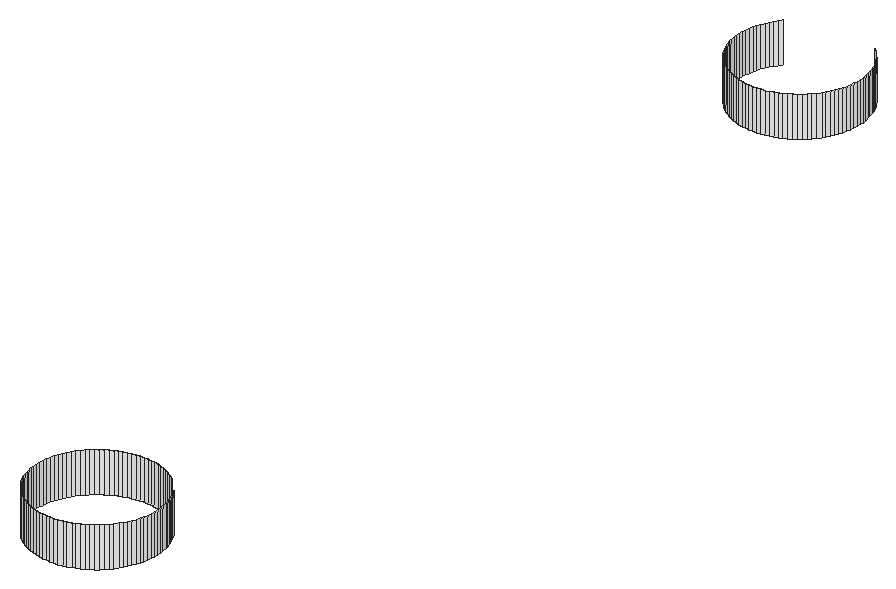
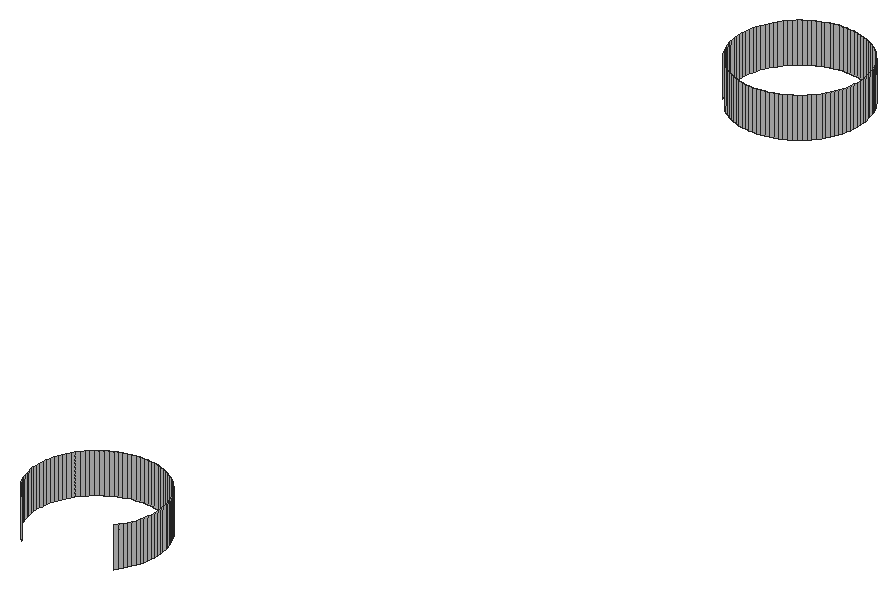
# SketchUp Ruby script. Lengths in inches.
U = 1.inch
M = Sketchup.active_model
def pt(a) = Geom::Point3d.new(a.map { |v| v * U })
def face(e, loops, mat)
  f = e.add_face(loops[0].map { |a| pt(a) })
  loops[1..].each { |l| e.add_face(l.map { |a| pt(a) }).erase! }
  f.material = f.back_material = mat if mat
  f
end
# faces: each face lists its corners as indices into pts; further lists are holes
def faces(e, pts, list, mat = nil) = list.each { |f| face(e, (f[0].is_a?(Array) ? f : [f]).map { |l| l.map { |i| pts[i] } }, mat) }
# xy, xz, yz: faces in a plane at the given z, y or x. An outline is a flat list of corners, or four numbers for a rectangle; further outlines are holes
def ring(l) = l.size == 4 ? [[l[0], l[1]], [l[2], l[1]], [l[2], l[3]], [l[0], l[3]]] : l.each_slice(2).to_a
def flat(e, list, mat, &to3) = list.each { |f| face(e, (f[0].is_a?(Array) ? f : [f]).map { |l| ring(l).map { |u, v| to3.(u, v) } }, mat) }
def xy(e, z, list, mat = nil) = flat(e, list, mat) { |x, y| [x, y, z] }
def xz(e, y, list, mat = nil) = flat(e, list, mat) { |x, z| [x, y, z] }
def yz(e, x, list, mat = nil) = flat(e, list, mat) { |y, z| [x, y, z] }
def lines(e, pts, list) = list.each { |a, b| e.add_line(pt(pts[a]), pt(pts[b])) }
# prism: a flat outline (further loops are holes) pulled along v
def prism(e, loops, v, mat = nil)
  f = face(e, loops, mat); d = Geom::Vector3d.new(v.map { |x| x * U })
  f.pushpull(f.normal.samedirection?(d) ? d.length : -d.length)
end
def box(e, o, s, mat = nil) = prism(e, [[o, [o[0] + s[0], o[1], o[2]], [o[0] + s[0], o[1] + s[1], o[2]], [o[0], o[1] + s[1], o[2]]]], [0, 0, s[2]], mat)
def at(x, y, z, deg = 0) = Geom::Transformation.translation(pt([x, y, z])) * Geom::Transformation.rotation(ORIGIN, Z_AXIS, deg.degrees)
def axes(o, x, y, z) = Geom::Transformation.new([*x, 0, *y, 0, *z, 0, *pt(o).to_a, 1])
def part(name) = M.definitions.add(name)
# library, detail: a bought-in or finely detailed component or shape, given as its bounding box
def library(name, o, s) = part(name).tap { |d| box(d.entities, o, s) }
def detail(e, o, s) = box(e.add_group.entities, o, s)
def put(e, d, t, mat = nil) = e.add_instance(d, t).tap { |i| i.material = mat if mat }
def group(e, t, mat = nil) = e.add_group.tap { |g| g.transformation = t; g.material = mat if mat }.entities
root = M.entities
M.materials.add("[Color M00]").color = [255, 255, 255]
xz(root,61,[[127.87,120,128.0625,122]],"[Color M00]")
xz(root,67,[[127.9375,120,128.13,122]],"[Color M00]")
xz(root,105,[[127.87,120,128.0625,122]],"[Color M00]")
yz(root,125,[[63.9375,120,64.13,122],[107.9375,120,108.13,122]],"[Color M00]")
yz(root,131,[[63.87,120,64.0625,122],[107.87,120,108.0625,122]],"[Color M00]")
p = [[127.5,61.04,120],[127.3125,61.08,120],[127.3125,61.08,122],[127.5,61.04,122],[127.68,61.02,120],[127.68,61.02,122],
  [127.87,61,120],[127.87,61,122],[128.25,61.01,120],[128.0625,61,120],[128.0625,61,122],[128.25,61.01,122],
  [128.4375,61.03,120],[128.4375,61.03,122],[128.62,61.07,120],[128.62,61.07,122],[127.13,61.13,120],[126.95,61.1875,120],
  [126.95,61.1875,122],[127.13,61.13,122],[128.81,61.11,120],[128.81,61.11,122],[128.98,61.17,120],[128.98,61.17,122],
  [126.78,61.26,120],[126.78,61.26,122],[129.16,61.23,120],[129.16,61.23,122],[129.33,61.3125,120],[129.33,61.3125,122],
  [126.61,61.34,120],[126.44,61.43,120],[126.44,61.43,122],[126.61,61.34,122],[129.5,61.4,120],[129.5,61.4,122],
  [126.29,61.54,120],[126.29,61.54,122],[129.66,61.5,120],[129.66,61.5,122],[126.14,61.65,120],[126.14,61.65,122],
  [129.8125,61.61,120],[129.8125,61.61,122],[125.99,61.77,120],[125.99,61.77,122],[129.96,61.73,120],[129.96,61.73,122],
  [130.1,61.86,120],[130.1,61.86,122],[125.86,61.9,120],[125.86,61.9,122],[125.73,62.04,120],[125.73,62.04,122],
  [130.23,61.99,120],[130.23,61.99,122],[125.61,62.1875,120],[125.61,62.1875,122],[130.35,62.14,120],[130.35,62.14,122],
  [130.46,62.29,120],[130.46,62.29,122],[125.5,62.34,120],[125.5,62.34,122],[125.4,62.5,120],[125.4,62.5,122],
  [130.57,62.44,120],[130.57,62.44,122],[130.66,62.61,120],[130.66,62.61,122],[125.3125,62.67,120],[125.3125,62.67,122],
  [130.74,62.78,120],[130.74,62.78,122],[125.23,62.84,120],[125.23,62.84,122],[125.17,63.02,120],[125.17,63.02,122],
  [130.8125,62.95,120],[130.8125,62.95,122],[125.11,63.19,120],[125.11,63.19,122],[130.87,63.13,120],[130.87,63.13,122],
  [130.92,63.3125,120],[130.92,63.3125,122],[125.07,63.38,120],[125.07,63.38,122],[130.96,63.5,120],[130.96,63.5,122],
  [125.03,63.5625,120],[125.03,63.5625,122],[130.98,63.68,120],[130.98,63.68,122],[125.01,63.75,120],[125.01,63.75,122],
  [131,63.87,120],[131,63.87,122],[125,63.9375,120],[125,63.9375,122],[125,64.13,120],[125.02,64.32,120],
  [125.02,64.32,122],[125,64.13,122],[130.99,64.25,120],[131,64.0625,120],[131,64.0625,122],[130.99,64.25,122],
  [130.97,64.4375,120],[130.97,64.4375,122],[125.04,64.5,120],[125.04,64.5,122],[130.93,64.62,120],[130.93,64.62,122],
  [125.08,64.6875,120],[125.08,64.6875,122],[130.89,64.81,120],[130.89,64.81,122],[125.13,64.87,120],[125.13,64.87,122],
  [130.83,64.98,120],[130.83,64.98,122],[125.1875,65.05,120],[125.1875,65.05,122],[125.26,65.22,120],[125.26,65.22,122],
  [130.77,65.16,120],[130.77,65.16,122],[125.34,65.39,120],[125.34,65.39,122],[130.6875,65.33,120],[130.6875,65.33,122],
  [130.6,65.5,120],[130.6,65.5,122],[125.43,65.56,120],[125.43,65.56,122],[130.5,65.66,120],[130.5,65.66,122],
  [125.54,65.71,120],[125.54,65.71,122],[125.65,65.86,120],[125.65,65.86,122],[125.77,66.01,120],[125.77,66.01,122],
  [125.9,66.14,120],[125.9,66.14,122],[126.04,66.27,120],[126.04,66.27,122],[126.1875,66.39,120],[126.1875,66.39,122],
  [126.34,66.5,120],[126.34,66.5,122],[129.71,66.46,120],[129.86,66.35,120],[129.86,66.35,122],[129.71,66.46,122],
  [126.5,66.6,120],[126.5,66.6,122],[129.56,66.57,120],[129.56,66.57,122],[126.67,66.6875,120],[126.67,66.6875,122],
  [129.39,66.66,120],[129.39,66.66,122],[126.84,66.77,120],[126.84,66.77,122],[129.05,66.8125,120],[129.22,66.74,120],
  [129.22,66.74,122],[129.05,66.8125,122],[127.02,66.83,120],[127.02,66.83,122],[127.19,66.89,120],[127.19,66.89,122],
  [128.87,66.87,120],[128.87,66.87,122],[127.38,66.93,120],[127.38,66.93,122],[127.5625,66.97,120],[127.5625,66.97,122],
  [128.5,66.96,120],[128.6875,66.92,120],[128.6875,66.92,122],[128.5,66.96,122],[127.75,66.99,120],[127.75,66.99,122],
  [127.9375,67,120],[127.9375,67,122],[128.13,67,120],[128.32,66.98,120],[128.32,66.98,122],[128.13,67,122],
  [127.5,105.04,120],[127.3125,105.08,120],[127.3125,105.08,122],[127.5,105.04,122],[127.68,105.02,120],[127.68,105.02,122],
  [127.87,105,120],[127.87,105,122],[128.25,105.01,120],[128.0625,105,120],[128.0625,105,122],[128.25,105.01,122],
  [128.4375,105.03,120],[128.4375,105.03,122],[128.62,105.07,120],[128.62,105.07,122],[127.13,105.13,120],[126.95,105.1875,120],
  [126.95,105.1875,122],[127.13,105.13,122],[128.81,105.11,120],[128.81,105.11,122],[128.98,105.17,120],[128.98,105.17,122],
  [126.78,105.26,120],[126.78,105.26,122],[129.16,105.23,120],[129.16,105.23,122],[129.33,105.3125,120],[129.33,105.3125,122],
  [126.61,105.34,120],[126.44,105.43,120],[126.44,105.43,122],[126.61,105.34,122],[129.5,105.4,120],[129.5,105.4,122],
  [126.29,105.54,120],[126.29,105.54,122],[129.66,105.5,120],[129.66,105.5,122],[126.14,105.65,120],[126.14,105.65,122],
  [129.8125,105.61,120],[129.8125,105.61,122],[125.99,105.77,120],[125.99,105.77,122],[129.96,105.73,120],[129.96,105.73,122],
  [130.1,105.86,120],[130.1,105.86,122],[125.86,105.9,120],[125.86,105.9,122],[125.73,106.04,120],[125.73,106.04,122],
  [130.23,105.99,120],[130.23,105.99,122],[125.61,106.1875,120],[125.61,106.1875,122],[130.35,106.14,120],[130.35,106.14,122],
  [130.46,106.29,120],[130.46,106.29,122],[125.5,106.34,120],[125.5,106.34,122],[125.4,106.5,120],[125.4,106.5,122],
  [130.57,106.44,120],[130.57,106.44,122],[130.66,106.61,120],[130.66,106.61,122],[125.3125,106.67,120],[125.3125,106.67,122],
  [130.74,106.78,120],[130.74,106.78,122],[125.23,106.84,120],[125.23,106.84,122],[125.17,107.02,120],[125.17,107.02,122],
  [130.8125,106.95,120],[130.8125,106.95,122],[125.11,107.19,120],[125.11,107.19,122],[130.87,107.13,120],[130.87,107.13,122],
  [130.92,107.3125,120],[130.92,107.3125,122],[125.07,107.38,120],[125.07,107.38,122],[130.96,107.5,120],[130.96,107.5,122],
  [125.03,107.5625,120],[125.03,107.5625,122],[130.98,107.68,120],[130.98,107.68,122],[125.01,107.75,120],[125.01,107.75,122],
  [131,107.87,120],[131,107.87,122],[125,107.9375,120],[125,107.9375,122],[125,108.13,120],[125.02,108.32,120],
  [125.02,108.32,122],[125,108.13,122],[130.99,108.25,120],[131,108.0625,120],[131,108.0625,122],[130.99,108.25,122],
  [130.97,108.4375,120],[130.97,108.4375,122],[125.04,108.5,120],[125.04,108.5,122],[130.93,108.62,120],[130.93,108.62,122],
  [125.08,108.6875,120],[125.08,108.6875,122],[130.89,108.81,120],[130.89,108.81,122],[125.13,108.87,120],[125.13,108.87,122],
  [130.83,108.98,120],[130.83,108.98,122],[125.1875,109.05,120],[125.1875,109.05,122],[125.26,109.22,120],[125.26,109.22,122],
  [130.77,109.16,120],[130.77,109.16,122],[125.34,109.39,120],[125.34,109.39,122],[130.6875,109.33,120],[130.6875,109.33,122],
  [130.6,109.5,120],[130.6,109.5,122],[125.43,109.56,120],[125.43,109.56,122],[130.5,109.66,120],[130.5,109.66,122],
  [125.54,109.71,120],[125.54,109.71,122],[125.65,109.86,120],[125.65,109.86,122],[130.39,109.8125,120],[130.39,109.8125,122],
  [130.27,109.96,120],[130.27,109.96,122],[130.14,110.1,120],[130.14,110.1,122],[130.01,110.23,120],[130.01,110.23,122],
  [129.86,110.35,120],[129.86,110.35,122]]
faces(root,p,[[0,1,2,3],[4,0,3,5],[6,4,5,7],[8,9,10,11],[12,8,11,13],[14,12,13,15],[16,17,18,19],[1,16,19,2],
  [20,14,15,21],[22,20,21,23],[17,24,25,18],[26,22,23,27],[28,26,27,29],[30,31,32,33],[24,30,33,25],[34,28,29,35],
  [31,36,37,32],[38,34,35,39],[36,40,41,37],[42,38,39,43],[40,44,45,41],[46,42,43,47],[48,46,47,49],[44,50,51,45],
  [50,52,53,51],[54,48,49,55],[52,56,57,53],[58,54,55,59],[60,58,59,61],[56,62,63,57],[62,64,65,63],[66,60,61,67],
  [68,66,67,69],[64,70,71,65],[72,68,69,73],[70,74,75,71],[74,76,77,75],[78,72,73,79],[76,80,81,77],[82,78,79,83],
  [84,82,83,85],[80,86,87,81],[88,84,85,89],[86,90,91,87],[92,88,89,93],[90,94,95,91],[96,92,93,97],[94,98,99,95],
  [100,101,102,103],[104,105,106,107],[108,104,107,109],[101,110,111,102],[112,108,109,113],[110,114,115,111],[116,112,113,117],[114,118,119,115],
  [120,116,117,121],[118,122,123,119],[122,124,125,123],[126,120,121,127],[124,128,129,125],[130,126,127,131],[132,130,131,133],[128,134,135,129],
  [136,132,133,137],[134,138,139,135],[138,140,141,139],[140,142,143,141],[142,144,145,143],[144,146,147,145],[146,148,149,147],[148,150,151,149],
  [152,153,154,155],[150,156,157,151],[158,152,155,159],[156,160,161,157],[162,158,159,163],[160,164,165,161],[166,167,168,169],[167,162,163,168],
  [164,170,171,165],[170,172,173,171],[174,166,169,175],[172,176,177,173],[176,178,179,177],[180,181,182,183],[181,174,175,182],[178,184,185,179],
  [184,186,187,185],[188,189,190,191],[189,180,183,190],[192,193,194,195],[196,192,195,197],[198,196,197,199],[200,201,202,203],[204,200,203,205],
  [206,204,205,207],[208,209,210,211],[193,208,211,194],[212,206,207,213],[214,212,213,215],[209,216,217,210],[218,214,215,219],[220,218,219,221],
  [222,223,224,225],[216,222,225,217],[226,220,221,227],[223,228,229,224],[230,226,227,231],[228,232,233,229],[234,230,231,235],[232,236,237,233],
  [238,234,235,239],[240,238,239,241],[236,242,243,237],[242,244,245,243],[246,240,241,247],[244,248,249,245],[250,246,247,251],[252,250,251,253],
  [248,254,255,249],[254,256,257,255],[258,252,253,259],[260,258,259,261],[256,262,263,257],[264,260,261,265],[262,266,267,263],[266,268,269,267],
  [270,264,265,271],[268,272,273,269],[274,270,271,275],[276,274,275,277],[272,278,279,273],[280,276,277,281],[278,282,283,279],[284,280,281,285],
  [282,286,287,283],[288,284,285,289],[286,290,291,287],[292,293,294,295],[296,297,298,299],[300,296,299,301],[293,302,303,294],[304,300,301,305],
  [302,306,307,303],[308,304,305,309],[306,310,311,307],[312,308,309,313],[310,314,315,311],[314,316,317,315],[318,312,313,319],[316,320,321,317],
  [322,318,319,323],[324,322,323,325],[320,326,327,321],[328,324,325,329],[326,330,331,327],[330,332,333,331],[334,328,329,335],[336,334,335,337],
  [338,336,337,339],[340,338,339,341],[342,340,341,343]],"[Color M00]")
